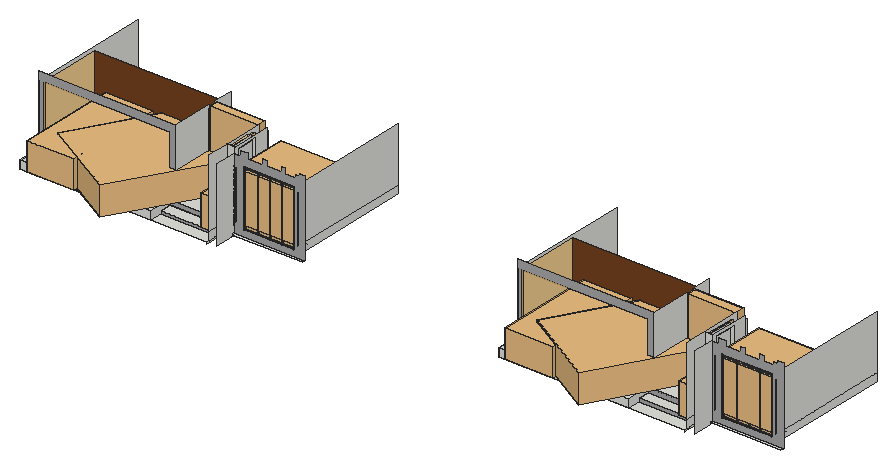
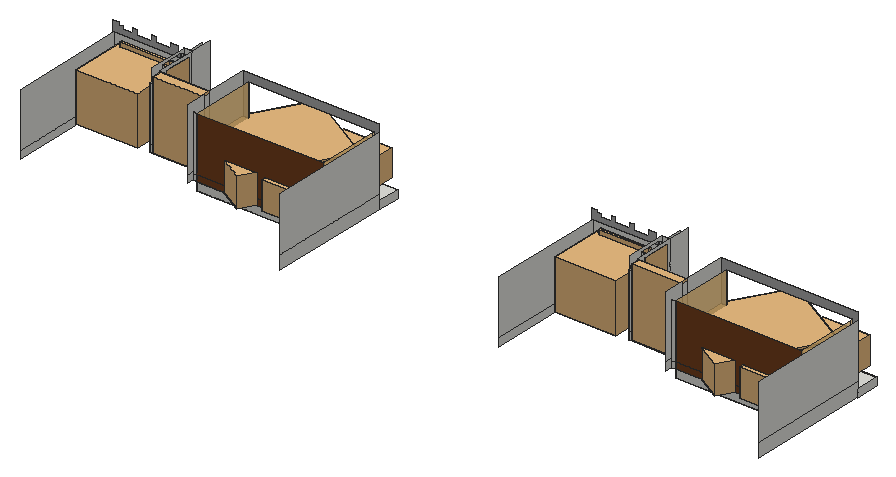
# SketchUp Ruby script. Lengths in inches.
U = 1.inch
M = Sketchup.active_model
def pt(a) = Geom::Point3d.new(a.map { |v| v * U })
def face(e, loops, mat)
  f = e.add_face(loops[0].map { |a| pt(a) })
  loops[1..].each { |l| e.add_face(l.map { |a| pt(a) }).erase! }
  f.material = f.back_material = mat if mat
  f
end
# faces: each face lists its corners as indices into pts; further lists are holes
def faces(e, pts, list, mat = nil) = list.each { |f| face(e, (f[0].is_a?(Array) ? f : [f]).map { |l| l.map { |i| pts[i] } }, mat) }
# xy, xz, yz: faces in a plane at the given z, y or x. An outline is a flat list of corners, or four numbers for a rectangle; further outlines are holes
def ring(l) = l.size == 4 ? [[l[0], l[1]], [l[2], l[1]], [l[2], l[3]], [l[0], l[3]]] : l.each_slice(2).to_a
def flat(e, list, mat, &to3) = list.each { |f| face(e, (f[0].is_a?(Array) ? f : [f]).map { |l| ring(l).map { |u, v| to3.(u, v) } }, mat) }
def xy(e, z, list, mat = nil) = flat(e, list, mat) { |x, y| [x, y, z] }
def xz(e, y, list, mat = nil) = flat(e, list, mat) { |x, z| [x, y, z] }
def yz(e, x, list, mat = nil) = flat(e, list, mat) { |y, z| [x, y, z] }
def lines(e, pts, list) = list.each { |a, b| e.add_line(pt(pts[a]), pt(pts[b])) }
# prism: a flat outline (further loops are holes) pulled along v
def prism(e, loops, v, mat = nil)
  f = face(e, loops, mat); d = Geom::Vector3d.new(v.map { |x| x * U })
  f.pushpull(f.normal.samedirection?(d) ? d.length : -d.length)
end
def box(e, o, s, mat = nil) = prism(e, [[o, [o[0] + s[0], o[1], o[2]], [o[0] + s[0], o[1] + s[1], o[2]], [o[0], o[1] + s[1], o[2]]]], [0, 0, s[2]], mat)
def at(x, y, z, deg = 0) = Geom::Transformation.translation(pt([x, y, z])) * Geom::Transformation.rotation(ORIGIN, Z_AXIS, deg.degrees)
def axes(o, x, y, z) = Geom::Transformation.new([*x, 0, *y, 0, *z, 0, *pt(o).to_a, 1])
def part(name) = M.definitions.add(name)
# library, detail: a bought-in or finely detailed component or shape, given as its bounding box
def library(name, o, s) = part(name).tap { |d| box(d.entities, o, s) }
def detail(e, o, s) = box(e.add_group.entities, o, s)
def put(e, d, t, mat = nil) = e.add_instance(d, t).tap { |i| i.material = mat if mat }
def group(e, t, mat = nil) = e.add_group.tap { |g| g.transformation = t; g.material = mat if mat }.entities
root = M.entities
M.materials.add("Glazing").color = [128, 128, 128]
M.materials["Glazing"].alpha = 0.05
M.materials.add("Powdercoating").color = [41, 44, 40]
M.materials.add("[Color M03]1").color = [170, 170, 170]
M.materials.add("[Wood Cherry Original]").color = [117, 66, 32]
M.materials.add("[Wood OSB]").color = [255, 207, 129]
M.materials["[Wood OSB]"].alpha = 0.8
c1 = library("plant1",[-367.84,-375.82,-125.45],[750.59,696.16,1346.74])
c2 = part("skp4FF")
put(c2.entities,c1,at(0,0,0))
c3 = part("Group\#15")
xy(c3.entities,0,[[0,-55.94,0.71,45.94]])
xy(c3.entities,0.2,[[0,-55.94,0.47,45.94],[0.47,45.94,0.71,46.42]])
xy(c3.entities,2.36,[[0.47,-55.94,0.71,46.42]])
xz(c3.entities,-55.94,[[0,0,0.71,0,0.71,2.36,0.47,2.36,0.47,0.2,0,0.2]])
xz(c3.entities,45.94,[[0,0,0.71,0.2]])
xz(c3.entities,46.42,[[0.47,0.2,0.71,2.36]])
yz(c3.entities,0,[[-55.94,0,45.94,0.2]])
yz(c3.entities,0.47,[[-55.94,0.2,46.42,2.36]])
yz(c3.entities,0.71,[[-55.94,0,45.94,0,45.94,0.2,46.42,0.2,46.42,2.36,-55.94,2.36]])
c4 = part("Group\#7")
xy(c4.entities,0,[[0,-59.09,0.71,45.94]])
xy(c4.entities,0.2,[[0,-59.09,0.47,45.94],[0.47,45.94,0.71,46.42]])
xy(c4.entities,2.36,[[0.47,-59.09,0.71,46.42]])
xz(c4.entities,-59.09,[[0,0,0.71,0,0.71,2.36,0.47,2.36,0.47,0.2,0,0.2]])
xz(c4.entities,45.94,[[0,0,0.71,0.2]])
xz(c4.entities,46.42,[[0.47,0.2,0.71,2.36]])
yz(c4.entities,0,[[-59.09,0,45.94,0.2]])
yz(c4.entities,0.47,[[-59.09,0.2,46.42,2.36]])
yz(c4.entities,0.71,[[-59.09,0,45.94,0,45.94,0.2,46.42,0.2,46.42,2.36,-59.09,2.36]])
c5 = part("Group\#16")
prism(c5.entities,[[[0.47,-56.18,0.2],[0,-56.18,0.2],[0,-56.18,0],[0.71,-56.18,0],[0.71,-56.18,2.36],[0.47,-56.18,2.36]]],[0,28.68,0])
c6 = part("Group\#10")
box(c6.entities,[-0.73,0,0],[27.99,0.55,102.05])
c7 = part("Group\#18")
xy(c7.entities,0,[[0.47,-56.18,0.47,-55.47,0,-55.47,0,-28.21,1.18,-28.21,1.18,-56.18]])
xy(c7.entities,0.2,[[0.71,-56.18,1.18,-28.21],[0,-55.47,0.47,-28.21],[0.47,-28.21,0.71,-27.74]])
xy(c7.entities,2.36,[[0.47,-56.18,0.71,-27.74]])
xz(c7.entities,-56.18,[[0.47,0,1.18,0,1.18,0.2,0.71,0.2,0.71,2.36,0.47,2.36]])
xz(c7.entities,-55.47,[[0,0,0.47,0.2]])
xz(c7.entities,-28.21,[[0,0,1.18,0.2]])
xz(c7.entities,-27.74,[[0.47,0.2,0.71,2.36]])
yz(c7.entities,0,[[-55.47,0,-28.21,0.2]])
yz(c7.entities,0.47,[[-56.18,0,-55.47,0.2],[-56.18,0.2,-27.74,2.36]])
yz(c7.entities,0.71,[[-56.18,0.2,-27.74,2.36]])
yz(c7.entities,1.18,[[-56.18,0,-28.21,0.2]])
c8 = part("Group\#34")
xy(c8.entities,0,[[-20.45,0,7.76,1.22]])
xy(c8.entities,0.06,[[-20.39,0.06,7.7,1.22]])
xy(c8.entities,0.47,[[-19.98,0,7.28,0.06]])
xy(c8.entities,101.89,[[-19.98,0,7.28,0.06]])
xy(c8.entities,102.3,[[-20.39,0.06,7.7,1.22]])
xy(c8.entities,102.36,[[-20.45,0,7.76,1.22]])
xz(c8.entities,0,[[[-20.45,0,7.76,102.36],[-19.98,0.47,7.28,101.89]]])
xz(c8.entities,0.06,[[[-20.39,0.06,7.7,102.3],[-19.98,0.47,7.28,101.89]]])
xz(c8.entities,1.22,[[[-20.45,0,7.76,102.36],[-20.39,0.06,7.7,102.3]]])
yz(c8.entities,-20.45,[[0,0,1.22,102.36]])
yz(c8.entities,-20.39,[[0.06,0.06,1.22,102.3]])
yz(c8.entities,-19.98,[[0,0.47,0.06,101.89]])
yz(c8.entities,7.28,[[0,0.47,0.06,101.89]])
yz(c8.entities,7.7,[[0.06,0.06,1.22,102.3]])
yz(c8.entities,7.76,[[0,0,1.22,102.36]])
c9 = part("Group\#6")
put(c9.entities,c3,axes([27.97,0,7.875],[1,0,0],[0,0,-1],[0,1,0]),"Powdercoating")
put(c9.entities,c4,axes([0.71,0,6.8],[-1,0,0],[0,0,-0.97687],[0,1,0]),"Powdercoating")
put(c9.entities,c5,axes([-27.5,0,-38.07],[0,0,-1],[-1,0,0],[0,1,0]),"Powdercoating")
put(c9.entities,c6,at(1.12,0.35,-38.39),"Glazing")
put(c9.entities,c7,axes([-27.5,0,63.35],[0,0,1],[-1,0,0],[0,1,0]),"Powdercoating")
put(c9.entities,c8,at(20.6875,1.0625,-38.54),"Powdercoating")
c10 = part("Component\#2")
put(c10.entities,c9,at(-1.18,4.5,38.86))
g1 = group(c10.entities,at(84.74,4.5,38.86))
put(g1,c3,axes([-27.97,0,7.875],[-1,0,0],[0,0,-1],[0,1,0]),"Powdercoating")
put(g1,c4,axes([-0.71,0,6.8],[1,0,0],[0,0,-0.97687],[0,1,0]),"Powdercoating")
put(g1,c5,axes([27.5,0,-38.07],[0,0,-1],[1,0,0],[0,1,0]),"Powdercoating")
put(g1,c6,axes([-1.12,0.35,-38.39],[-1,0,0],[0,1,0],[0,0,1]),"Glazing")
put(g1,c7,axes([27.5,0,63.35],[0,0,1],[1,0,0],[0,1,0]),"Powdercoating")
put(g1,c8,axes([-20.6875,1.0625,-38.54],[-1,0,0],[0,1,0],[0,0,1]),"Powdercoating")
g2 = group(c10.entities,at(56.0625,4.5,38.86))
put(g2,c3,axes([-27.97,0,7.875],[-1,0,0],[0,0,-1],[0,1,0]),"Powdercoating")
put(g2,c5,axes([27.5,0,-38.07],[0,0,-1],[1,0,0],[0,1,0]),"Powdercoating")
put(g2,c6,axes([-1.12,0.35,-38.39],[-1,0,0],[0,1,0],[0,0,1]),"Glazing")
put(g2,c7,axes([27.5,0,63.35],[0,0,1],[1,0,0],[0,1,0]),"Powdercoating")
put(g2,c8,axes([-20.6875,1.0625,-38.54],[-1,0,0],[0,1,0],[0,0,1]),"Powdercoating")
g3 = group(g2,at(-0.71,0,6.8),"Powdercoating")
xy(g3,-45.34,[[0.47,0.2,0.71,2.36]])
xy(g3,-44.88,[[0,0,0.71,0.2]])
xy(g3,57.73,[[0,0,0.71,0,0.71,2.36,0.47,2.36,0.47,0.2,0,0.2]])
xz(g3,0,[[0,-44.88,0.71,57.73]])
xz(g3,0.2,[[0.47,-45.34,0.71,-44.88],[0,-44.88,0.47,57.73]])
xz(g3,2.36,[[0.47,-45.34,0.71,57.73]])
yz(g3,0,[[0,-44.88,0.2,57.73]])
yz(g3,0.47,[[0.2,-45.34,2.36,57.73]])
yz(g3,0.71,[[0.2,-45.34,2.36,-45.34,2.36,57.73,0,57.73,0,-44.88,0.2,-44.88]])
put(c10.entities,c9,axes([-33.94,4.5,38.86],[1.14218,0,0],[0,1,0],[0,0,1]))
c11 = part("sliding door")
put(c11.entities,c10,at(0,-4.5,-0.08))
c12 = library("panneau+shadow+blanc+bourdon+naturel",[-47.99,-1.29,1.53],[97.82,5.86,114.18])
c13 = library("002+Bmw+M4+++mat3.4+2017",[-252.8,19.48,9.01],[196.94,171.32,55.15])
c14 = library("BMW 8 Series M850i 2019",[-14.25,0.77,-0.16],[87.38,190.63,50.87])
c15 = library("元件\#5",[-4.39,0,0],[5.37,35.83,90.55])
c16 = library("Group\#553",[0,0,0],[134.5,122.36,106.97])
c17 = library("modern+door",[0,0,0],[59.06,11.8125,86.61])
xy(root,-24.25,[[200.03,335.84,486.41,335.84,486.41,528.53,208.91,528.53,208.91,387.84,200.03,387.84],[486.41,335.84,609.09,362.97],[1248.34,335.84,1534.73,335.84,1534.73,528.53,1257.22,528.53,1257.22,387.84,1248.34,387.84],[1534.73,335.84,1657.41,362.97],[486.41,362.97,609.09,387.84],
  [1534.73,362.97,1657.41,387.84]])
xy(root,-22.8,[[626.68,381.72,782.78,387.84],[1674.99,381.72,1831.09,387.84]])
xy(root,-16.95,[[486.41,362.97,609.09,387.84],[1534.73,362.97,1657.41,387.84]])
xy(root,-9.875,[[647.46,387.84,757.46,394.91],[1695.77,387.84,1805.77,394.91]])
xy(root,-6.625,[[200.03,335.84,486.41,335.84,486.41,528.53,208.91,528.53,208.91,387.84,200.03,387.84],[1248.34,335.84,1534.73,335.84,1534.73,528.53,1257.22,528.53,1257.22,387.84,1248.34,387.84],[486.41,387.84,493.2,528.53],[499.53,387.84,609.09,387.84,609.09,398.1,615.97,398.1,615.97,448.72,609.09,448.72,609.09,477.09,607.63,477.09,607.63,494.59,500.81,494.59,500.81,477.09,499.53,477.09],[609.09,387.84,626.68,389.4],
  [1534.73,387.84,1541.52,528.53],[1547.84,387.84,1657.41,387.84,1657.41,398.1,1664.28,398.1,1664.28,448.72,1657.41,448.72,1657.41,477.09,1655.94,477.09,1655.94,494.59,1549.12,494.59,1549.12,477.09,1547.84,477.09],[1657.41,387.84,1674.99,389.4],[609.09,389.4,626.68,398.1],[1657.41,389.4,1674.99,398.1],
  [609.09,448.72,626.68,477.09],[1657.41,448.72,1674.99,477.09]])
xz(root,335.84,[[200.03,-24.25,486.41,-6.625],[1248.34,-24.25,1534.73,-6.625]])
xz(root,362.97,[[486.41,-24.25,609.09,-16.95],[1534.73,-24.25,1657.41,-16.95]],"[Color M03]1")
xz(root,387.84,[[609.09,-27.66,626.68,-22.8],[1657.41,-27.66,1674.99,-22.8],[200.03,-24.25,208.91,-22.8],[486.41,-24.25,609.09,-22.8],[1248.34,-24.25,1257.22,-22.8],
  [1534.73,-24.25,1657.41,-22.8],[200.03,-22.8,208.91,-6.625],[486.41,-22.8,609.09,-16.95],[609.09,-22.8,626.68,-6.625],[1248.34,-22.8,1257.22,-6.625],
  [1534.73,-22.8,1657.41,-16.95],[1657.41,-22.8,1674.99,-6.625]])
xz(root,387.84,[[[626.68,-22.8,782.78,-22.8,782.78,144.3125,771.49,144.3125,771.49,139.5,761.74,139.5,761.74,133.625,739.28,133.625,739.28,144.3125,730.86,144.3125,730.86,133.625,698.65,133.625,698.65,144.3125,689.24,144.3125,689.24,133.625,657.03,133.625,657.03,144.3125,641.55,144.3125,641.55,133.625,626.68,133.625],[647.46,-9.875,757.46,115.81]],[[1674.99,-22.8,1831.09,-22.8,1831.09,144.3125,1819.8,144.3125,1819.8,139.5,1810.05,139.5,1810.05,133.625,1787.59,133.625,1787.59,144.3125,1779.17,144.3125,1779.17,133.625,1746.96,133.625,1746.96,144.3125,1737.55,144.3125,1737.55,133.625,1705.34,133.625,1705.34,144.3125,1689.86,144.3125,1689.86,133.625,1674.99,133.625],[1695.77,-9.875,1805.77,115.81]],[486.41,-16.95,609.09,-6.625],[1534.73,-16.95,1657.41,-6.625],[200.03,-6.625,208.91,6.75],
  [486.41,-6.625,499.53,-6.625,499.53,144.3125,497.6,144.3125,497.6,144.9375,200.03,144.9375,200.03,6.75,208.91,6.75,208.91,126.75,486.41,126.75],[1248.34,-6.625,1257.22,6.75],[1534.73,-6.625,1547.84,-6.625,1547.84,144.3125,1545.92,144.3125,1545.92,144.9375,1248.34,144.9375,1248.34,6.75,1257.22,6.75,1257.22,126.75,1534.73,126.75]],"[Color M03]1")
xz(root,389.4,[[609.09,-6.625,626.68,144.9375],[1657.41,-6.625,1674.99,144.9375]])
xz(root,394.91,[[616.45,-9.875,647.46,6.75],[757.46,-9.875,775.16,6.75],[1664.77,-9.875,1695.77,6.75],[1805.77,-9.875,1823.47,6.75],[616.45,6.75,616.45,126.75,775.16,126.75,775.16,6.75,757.46,6.75,757.46,115.81,647.46,115.81,647.46,6.75],
  [1664.77,6.75,1664.77,126.75,1823.47,126.75,1823.47,6.75,1805.77,6.75,1805.77,115.81,1695.77,115.81,1695.77,6.75]])
xz(root,398.1,[[609.09,-6.625,615.97,138.5625],[615.97,-6.625,626.68,138.5625],[1657.41,-6.625,1664.28,138.5625],[1664.28,-6.625,1674.99,138.5625]])
xz(root,448.72,[[609.09,-6.625,615.97,138.5625],[615.97,-6.625,626.68,138.5625],[1657.41,-6.625,1664.28,138.5625],[1664.28,-6.625,1674.99,138.5625]])
xz(root,477.09,[[499.53,-6.625,500.81,6.75],[607.63,-6.625,609.09,6.75],[609.09,-6.625,626.68,6.75],[1547.84,-6.625,1549.12,6.75],[1655.94,-6.625,1657.41,6.75],
  [1657.41,-6.625,1674.99,6.75],[499.53,6.75,500.81,126.75],[607.63,6.75,609.09,126.75],[609.09,6.75,626.68,126.75],[1547.84,6.75,1549.12,126.75],
  [1655.94,6.75,1657.41,126.75],[1657.41,6.75,1674.99,126.75]])
xz(root,494.59,[[499.53,-9.875,500.81,6.75],[500.81,-9.875,607.63,-6.625],[607.63,-9.875,616.45,6.75],[1547.84,-9.875,1549.12,6.75],[1549.12,-9.875,1655.94,-6.625],
  [1655.94,-9.875,1664.77,6.75],[499.53,6.75,500.81,126.75],[607.63,6.75,616.45,126.75],[1547.84,6.75,1549.12,126.75],[1655.94,6.75,1664.77,126.75]])
xz(root,528.53,[[208.91,-24.25,262.79,-6.625],[262.79,-24.25,486.41,-6.625],[1257.22,-24.25,1311.1,-6.625],[1311.1,-24.25,1534.73,-6.625],[486.41,-6.625,493.2,6.75],
  [1534.73,-6.625,1541.52,6.75],[486.41,6.75,493.2,126.75],[1534.73,6.75,1541.52,126.75]])
xz(root,528.53,[[208.91,-6.625,262.79,6.75],[262.79,-6.625,486.41,6.75],[1257.22,-6.625,1311.1,6.75],[1311.1,-6.625,1534.73,6.75],[208.91,6.75,486.41,126.75],
  [1257.22,6.75,1534.73,126.75]],"[Wood Cherry Original]")
xz(root,538.16,[[208.91,-9.875,262.79,6.75]])
yz(root,200.03,[[335.84,-24.25,387.84,-6.625],[387.84,-22.8,659.09,6.75],[387.84,6.75,659.09,126.75]])
yz(root,208.91,[[387.84,-24.25,394.91,-6.625],[394.91,-24.25,528.53,-6.625]])
yz(root,208.91,[[387.84,-6.625,394.91,126.75],[394.91,-6.625,528.53,126.75]],"[Wood OSB]")
yz(root,486.41,[[335.84,-24.25,362.97,-24.25,362.97,-16.95,387.84,-16.95,387.84,-6.625,335.84,-6.625],[362.97,-24.25,364.46,-24.25,364.46,-16.95,362.97,-17.6],[364.46,-24.25,387.84,-16.95],[387.84,-24.25,394.91,-6.625],[394.91,-24.25,528.53,-6.625],
  [362.97,-17.6,364.46,-16.95,362.97,-16.95]])
yz(root,486.41,[[387.84,-6.625,528.53,126.75]],"[Wood OSB]")
yz(root,499.53,[[494.59,-9.875,538.16,6.75],[387.84,-6.625,477.09,6.75],[387.84,6.75,477.09,144.3125],[494.59,6.75,538.16,144.3125]])
yz(root,500.81,[[477.09,-6.625,494.59,6.75],[477.09,6.75,494.59,138]])
yz(root,607.63,[[477.09,-6.625,494.59,138]])
yz(root,609.09,[[335.84,-27.66,341.03,-24.25],[341.03,-27.66,362.97,-24.25],[362.97,-27.66,387.84,-24.25],[341.03,-24.25,341.03,-6.625,387.84,-6.625,387.84,-16.95,362.97,-16.95,362.97,-24.25],[362.97,-24.25,387.84,-16.95],
  [341.03,-6.625,341.03,144.9375,365.47,144.9375,365.47,144.3125,389.4,144.3125,389.4,-6.625],[389.4,-6.625,389.4,144.3125,477.09,144.3125,477.09,-6.625,448.72,-6.625,448.72,138.5625,398.1,138.5625,398.1,-6.625]])
yz(root,615.97,[[398.1,-6.625,448.72,138.5625]])
yz(root,616.45,[[394.91,-9.875,494.59,6.75],[394.91,6.75,494.59,126.75]])
yz(root,626.68,[[341.03,-27.66,381.72,-27.66,381.72,-22.8,387.84,-22.8,387.84,133.625,341.03,133.625],[381.72,-27.66,387.84,-22.8],[387.84,-6.625,389.4,133.625],[389.4,-6.625,398.1,-6.625,398.1,138.5625,448.72,138.5625,448.72,-6.625,477.09,-6.625,477.09,144.3125,389.4,144.3125]])
yz(root,647.46,[[387.84,-9.875,394.91,6.75],[387.84,6.75,394.91,115.81]])
yz(root,757.46,[[387.84,-9.875,394.91,6.75],[387.84,6.75,394.91,115.81]])
yz(root,775.16,[[394.91,-9.875,652.02,6.75],[394.91,6.75,652.02,126.75]])
yz(root,1248.34,[[335.84,-24.25,387.84,-6.625],[387.84,-22.8,659.09,6.75],[387.84,6.75,659.09,126.75]])
yz(root,1257.22,[[387.84,-24.25,394.91,-6.625],[394.91,-24.25,528.53,-6.625]])
yz(root,1257.22,[[387.84,-6.625,394.91,126.75],[394.91,-6.625,528.53,126.75]],"[Wood OSB]")
yz(root,1534.73,[[335.84,-24.25,362.97,-24.25,362.97,-16.95,387.84,-16.95,387.84,-6.625,335.84,-6.625],[362.97,-24.25,364.46,-24.25,364.46,-16.95,362.97,-17.6],[364.46,-24.25,387.84,-16.95],[387.84,-24.25,394.91,-6.625],[394.91,-24.25,528.53,-6.625],
  [362.97,-17.6,364.46,-16.95,362.97,-16.95]])
yz(root,1534.73,[[387.84,-6.625,528.53,126.75]],"[Wood OSB]")
yz(root,1547.84,[[494.59,-9.875,538.16,6.75],[387.84,-6.625,477.09,6.75],[387.84,6.75,477.09,144.3125],[494.59,6.75,538.16,144.3125]])
yz(root,1549.12,[[477.09,-6.625,494.59,6.75],[477.09,6.75,494.59,138]])
yz(root,1655.94,[[477.09,-6.625,494.59,138]])
yz(root,1657.41,[[335.84,-27.66,341.03,-24.25],[341.03,-27.66,362.97,-24.25],[362.97,-27.66,387.84,-24.25],[341.03,-24.25,341.03,-6.625,387.84,-6.625,387.84,-16.95,362.97,-16.95,362.97,-24.25],[362.97,-24.25,387.84,-16.95],
  [341.03,-6.625,341.03,144.9375,365.47,144.9375,365.47,144.3125,389.4,144.3125,389.4,-6.625],[389.4,-6.625,389.4,144.3125,477.09,144.3125,477.09,-6.625,448.72,-6.625,448.72,138.5625,398.1,138.5625,398.1,-6.625]])
yz(root,1664.28,[[398.1,-6.625,448.72,138.5625]])
yz(root,1664.77,[[394.91,-9.875,494.59,6.75],[394.91,6.75,494.59,126.75]])
yz(root,1674.99,[[341.03,-27.66,381.72,-27.66,381.72,-22.8,387.84,-22.8,387.84,133.625,341.03,133.625],[381.72,-27.66,387.84,-22.8],[387.84,-6.625,389.4,133.625],[389.4,-6.625,398.1,-6.625,398.1,138.5625,448.72,138.5625,448.72,-6.625,477.09,-6.625,477.09,144.3125,389.4,144.3125]])
yz(root,1695.77,[[387.84,-9.875,394.91,6.75],[387.84,6.75,394.91,115.81]])
yz(root,1805.77,[[387.84,-9.875,394.91,6.75],[387.84,6.75,394.91,115.81]])
yz(root,1823.47,[[394.91,-9.875,652.02,6.75],[394.91,6.75,652.02,126.75]])
p = [[262.79,538.16,6.75],[262.79,528.53,6.75],[609.09,387.84,6.75],[626.68,387.84,6.75],[782.78,394.91,6.75],[775.16,394.91,6.75],
  [1831.09,394.91,6.75],[1823.47,394.91,6.75],[1311.1,538.16,6.75],[1311.1,528.53,6.75],[1657.41,387.84,6.75],[1674.99,387.84,6.75]]
lines(root,p,[[0,1],[2,3],[4,5],[6,7],[8,9],[10,11]])
put(root,c2,axes([595.24,377.53,-10.1],[0.04953,0,0],[0,0.04953,0],[0,0,0.04953]))
put(root,c2,axes([1643.55,377.53,-10.1],[0.04953,0,0],[0,0.04953,0],[0,0,0.04953]))
put(root,c11,axes([680.24,389.625,-9.875],[0.91114,0,0],[0,0.755,0],[0,0,1.2092]))
put(root,c11,axes([1728.56,389.625,-9.875],[0.91114,0,0],[0,0.755,0],[0,0,1.2092]))
put(root,c12,axes([701.43,396.2,-11.56],[1.12452,0,0],[0,1,0],[0,0,1.10083]))
put(root,c12,axes([1749.74,396.2,-11.56],[1.12452,0,0],[0,1,0],[0,0,1.10083]))
put(root,c13,axes([596.27,505.88,-16.98],[0.575,0.99593,0],[-0.99593,0.575,0],[0,0,1.15]))
put(root,c13,axes([1644.58,505.88,-16.98],[0.575,0.99593,0],[-0.99593,0.575,0],[0,0,1.15]))
put(root,c14,axes([320.38,539.85,-6.43],[-1.19,0,0],[0,-1.19,0],[0,0,1.19]))
put(root,c14,axes([1368.69,539.85,-6.43],[-1.19,0,0],[0,-1.19,0],[0,0,1.19]))
put(root,c15,axes([612.9375,400.79,-6.625],[1.43,0,0],[0,1.6588,0],[0,0,1.6016]))
put(root,c15,axes([1661.25,400.79,-6.625],[1.43,0,0],[0,1.6588,0],[0,0,1.6016]))
put(root,c16,at(766.26,510.2,0.1,-180))
put(root,c16,at(1814.58,510.2,0.1,-180))
put(root,c17,axes([501.55,476.89,-6.625],[1.79618,0,0],[0,1.7271,0],[0,0,1.7271]))
put(root,c17,axes([1549.87,476.89,-6.625],[1.79618,0,0],[0,1.7271,0],[0,0,1.7271]))
